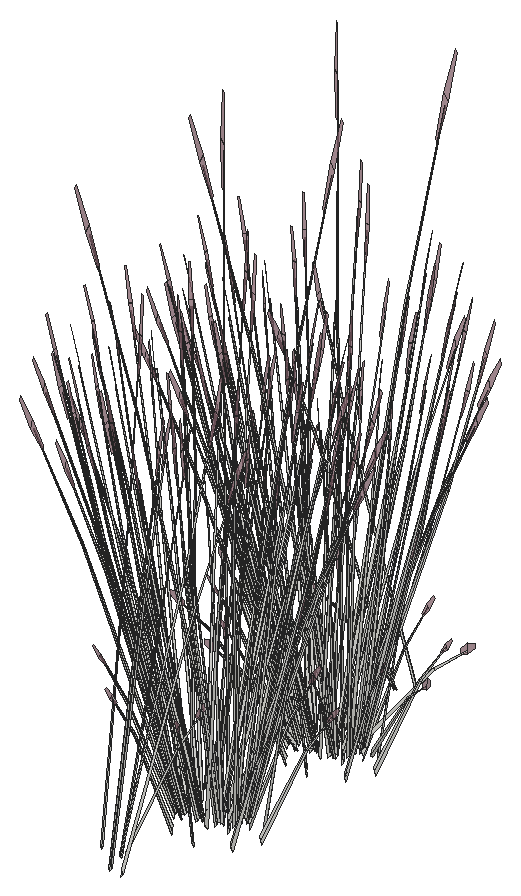
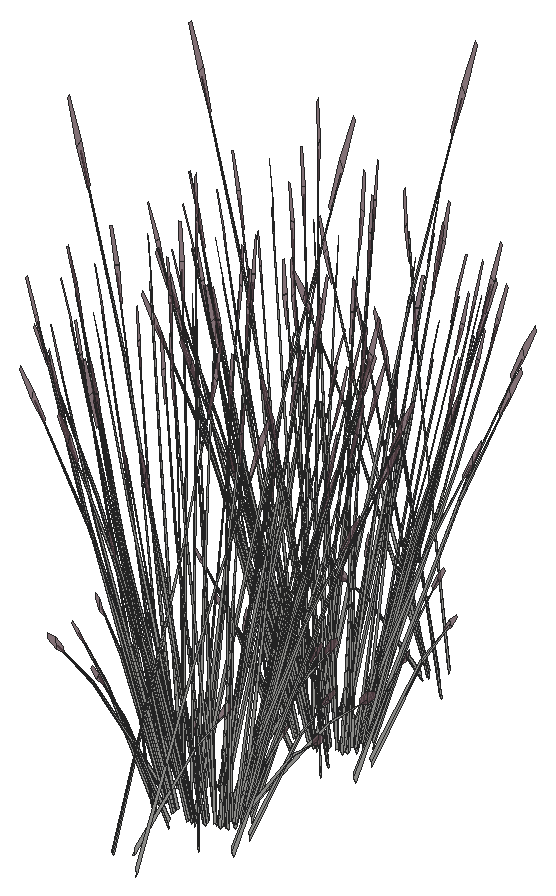
# SketchUp Ruby script. Lengths in inches.
U = 1.inch
M = Sketchup.active_model
def pt(a) = Geom::Point3d.new(a.map { |v| v * U })
def face(e, loops, mat)
  f = e.add_face(loops[0].map { |a| pt(a) })
  loops[1..].each { |l| e.add_face(l.map { |a| pt(a) }).erase! }
  f.material = f.back_material = mat if mat
  f
end
# faces: each face lists its corners as indices into pts; further lists are holes
def faces(e, pts, list, mat = nil) = list.each { |f| face(e, (f[0].is_a?(Array) ? f : [f]).map { |l| l.map { |i| pts[i] } }, mat) }
# xy, xz, yz: faces in a plane at the given z, y or x. An outline is a flat list of corners, or four numbers for a rectangle; further outlines are holes
def ring(l) = l.size == 4 ? [[l[0], l[1]], [l[2], l[1]], [l[2], l[3]], [l[0], l[3]]] : l.each_slice(2).to_a
def flat(e, list, mat, &to3) = list.each { |f| face(e, (f[0].is_a?(Array) ? f : [f]).map { |l| ring(l).map { |u, v| to3.(u, v) } }, mat) }
def xy(e, z, list, mat = nil) = flat(e, list, mat) { |x, y| [x, y, z] }
def xz(e, y, list, mat = nil) = flat(e, list, mat) { |x, z| [x, y, z] }
def yz(e, x, list, mat = nil) = flat(e, list, mat) { |y, z| [x, y, z] }
def lines(e, pts, list) = list.each { |a, b| e.add_line(pt(pts[a]), pt(pts[b])) }
# prism: a flat outline (further loops are holes) pulled along v
def prism(e, loops, v, mat = nil)
  f = face(e, loops, mat); d = Geom::Vector3d.new(v.map { |x| x * U })
  f.pushpull(f.normal.samedirection?(d) ? d.length : -d.length)
end
def box(e, o, s, mat = nil) = prism(e, [[o, [o[0] + s[0], o[1], o[2]], [o[0] + s[0], o[1] + s[1], o[2]], [o[0], o[1] + s[1], o[2]]]], [0, 0, s[2]], mat)
def at(x, y, z, deg = 0) = Geom::Transformation.translation(pt([x, y, z])) * Geom::Transformation.rotation(ORIGIN, Z_AXIS, deg.degrees)
def axes(o, x, y, z) = Geom::Transformation.new([*x, 0, *y, 0, *z, 0, *pt(o).to_a, 1])
def part(name) = M.definitions.add(name)
# library, detail: a bought-in or finely detailed component or shape, given as its bounding box
def library(name, o, s) = part(name).tap { |d| box(d.entities, o, s) }
def detail(e, o, s) = box(e.add_group.entities, o, s)
def put(e, d, t, mat = nil) = e.add_instance(d, t).tap { |i| i.material = mat if mat }
def group(e, t, mat = nil) = e.add_group.tap { |g| g.transformation = t; g.material = mat if mat }.entities
root = M.entities
M.materials.add("LightPink_Translucent").color = [144, 107, 117]
M.materials["LightPink_Translucent"].alpha = 0.75
c1 = part("blade")
p = [[2.15,0.21,22],[0,0.17,0],[0.09,0.45,0],[2.18,0.31,22],[2.29,0.31,22],[0.38,0.45,0],
  [2.48,0.24,33],[2.49,0.24,33],[2.48,0.22,33]]
faces(c1.entities,p,[[0,1,2,3],[4,5,2,3],[6,3,4,7],[8,0,3,6]])
c2 = part("seeds")
p = [[0.3,-0.1,1.38],[-0.01,-0.03,1.59],[-0.01,-0.03,0.03],[0.14,-0.07,-0.07],[0.29,-0.03,3],[0.15,0.01,3.11]]
faces(c2.entities,p,[[0,1,2,3],[1,0,4,5]],"LightPink_Translucent")
c3 = part("blade with seeds")
put(c3.entities,c1,at(0,0,0))
put(c3.entities,c2,axes([2.4,0.25,30.99],[1.5799,-0.05474,1.17369],[-0.12525,1.92788,0.29478],[-0.07173,-0.02425,1.56792]))
put(root,c3,axes([333.96,337.15,51.43],[-0.11542,-0.12546,1.51428],[0.53333,-0.10562,0.12244],[0.12054,0.19696,0.64734]))
put(root,c3,axes([333.45,338.05,52],[-0.15222,0.30049,-0.31292],[-0.44409,-0.08764,0.40398],[0.04072,0.12098,0.77298]))
put(root,c3,axes([332.49,337.47,52.72],[-0.01314,0.36145,-0.69681],[-0.55324,-0.02428,0.08409],[-0.05838,0.15313,0.9857]))
put(root,c3,axes([333.02,337.21,51.43],[-0.01236,-0.14998,1.51428],[0.53562,0.09949,0.12244],[-0.03313,0.21373,0.64734]))
put(root,c3,axes([333.5,337.78,52.4],[0.24099,0.31773,-0.62776],[-0.49607,0.17707,0.07576],[0.05635,0.15352,0.88802]))
put(root,c3,axes([333.14,338.58,52.17],[0.064,0.06292,1.54581],[0.51651,0.02472,-0.24447],[0.05194,0.13877,0.12397]))
put(root,c3,axes([332.69,344.625,51.43],[0.11542,0.12546,1.51428],[-0.53333,0.10562,0.12244],[-0.12054,-0.19696,0.64734]))
put(root,c3,axes([334.11,344.72,52.4],[-0.24099,-0.31773,-0.62776],[0.49607,-0.17707,0.07576],[-0.05635,-0.15352,0.88802]))
put(root,c3,axes([332.31,337.98,50.97],[0.01109,-0.20172,1.3638],[0.49896,0.10655,0.18846],[-0.04323,0.21498,0.64398]))
put(root,c3,axes([335.12,345.03,52.4],[0.01314,-0.36145,-0.62776],[0.55324,0.02428,0.07576],[0.05838,-0.15313,0.88802]))
put(root,c3,axes([334.16,344.45,52],[0.15222,-0.30049,-0.31292],[0.44409,0.08764,0.40398],[-0.04072,-0.12098,0.77298]))
put(root,c3,axes([334.5,344.85,51.43],[-0.09401,0.13431,1.51428],[-0.3944,-0.27795,0.12244],[0.17792,-0.17323,0.64734]))
put(root,c3,axes([333.93,344.66,52.14],[-0.49634,-0.09796,-0.45151],[0.17013,-0.33585,-0.34973],[-0.04551,-0.13522,0.86392]))
put(root,c3,axes([334.24,343.82,50.44],[0.06477,0.22786,1.01491],[-0.35932,-0.1262,0.74569],[0.03867,-0.11667,0.22354]))
put(root,c3,axes([335.01,344.91,52.14],[-0.36145,-0.26255,-0.45151],[0.38183,-0.22994,-0.34973],[0.055,-0.1334,0.86392]))
put(root,c3,axes([334.36,344.64,52.45],[-0.49409,0.18193,-0.10745],[-0.24281,-0.32289,-0.59638],[-0.06519,-0.13607,0.90619]))
put(root,c3,axes([335.38,345.05,52.45],[-0.55492,-0.01936,-0.10745],[0.01517,-0.36657,-0.59638],[0.03855,-0.14118,0.90619]))
put(root,c3,axes([335.35,344.8125,52],[0.34164,-0.20573,-0.31292],[0.3234,0.23491,0.40398],[0.04921,-0.11936,0.77298]))
put(root,c3,axes([332.39,344.09,50.44],[0.26338,0.136,1.01491],[-0.38358,0.08175,0.74569],[-0.08207,-0.10452,0.22354]))
put(root,c3,axes([333.03,344.81,52.4],[-0.43054,-0.18887,-0.62776],[0.30598,-0.33097,0.07576],[-0.15599,-0.11277,0.88802]))
put(root,c3,axes([332.88,344.56,52],[-0.07798,-0.31474,-0.31292],[0.44579,-0.08311,0.40398],[-0.11974,-0.09019,0.77298]))
put(root,c3,axes([331.92,345.02,51.43],[0.18755,0.06732,1.51428],[-0.38813,0.28243,0.12244],[-0.24191,-0.12741,0.64734]))
put(root,c3,axes([332.83,344.82,52.14],[-0.49824,0.09289,-0.45151],[-0.08716,-0.35177,-0.34973],[-0.13382,-0.10081,0.86392]))
put(root,c3,axes([335.77,345.66,52.4],[0.26374,-0.30832,-0.62776],[0.46217,0.21911,0.07576],[0.15748,-0.11171,0.88802]))
put(root,c3,axes([335.76,345.52,52.14],[-0.12971,-0.3568,-0.45151],[0.49122,-0.06241,-0.34973],[0.14077,-0.09583,0.86392]))
put(root,c3,axes([335.99,345.77,52.45],[-0.46706,-0.21546,-0.10745],[0.26908,-0.31203,-0.59638],[0.13196,-0.10846,0.90619]))
put(root,c3,axes([334.06,346.95,50.9375],[0.43633,0.15757,1.33654],[-0.42745,0.33945,0.52853],[-0.19146,-0.20119,1.12046]))
put(root,c3,axes([336.36,344.81,50.44],[-0.16818,0.19891,1.01491],[-0.14456,-0.26725,0.74569],[0.1389,-0.06697,0.22354]))
put(root,c3,axes([336.12,345.55,52],[0.43951,-0.05584,-0.31292],[0.11606,0.31924,0.40398],[0.12595,-0.08575,0.77298]))
put(root,c3,axes([331.85,345.11,52],[-0.28729,-0.24465,-0.31292],[0.32804,-0.23159,0.40398],[-0.16667,-0.03524,0.77298]))
put(root,c3,axes([332.15,345.28,52.4],[-0.50473,-0.00941,-0.62776],[0.0339,-0.39618,0.07576],[-0.21383,-0.04181,0.88802]))
put(root,c3,axes([331.98,345.36,52.14],[-0.36663,0.25884,-0.45151],[-0.32109,-0.27343,-0.34973],[-0.18628,-0.03938,0.86392]))
put(root,c3,axes([331.16,345.7,50.44],[0.32236,-0.02796,1.01491],[-0.20448,0.24636,0.74569],[-0.1593,-0.03696,0.22354]))
put(root,c3,axes([332.18,345.09,52.45],[-0.02704,0.39739,-0.10745],[-0.51189,-0.01086,-0.59638],[-0.19715,-0.0276,0.90619]))
put(root,c3,axes([336.01,346.61,52.45],[-0.25405,-0.35383,-0.10745],[0.45089,-0.17388,-0.59638],[0.19001,-0.04668,0.90619]))
put(root,c3,axes([335.98,346.31,52.14],[0.13679,-0.35544,-0.45151],[0.46898,0.12183,-0.34973],[0.18882,-0.03259,0.86392]))
put(root,c3,axes([331.52,345.63,51.43],[0.20943,-0.00885,1.51428],[-0.13893,0.38357,0.12244],[-0.29846,-0.02372,0.64734]))
put(root,c3,axes([335.9,346.4375,52.4],[0.44368,-0.17257,-0.62776],[0.24726,0.35524,0.07576],[0.21437,-0.04035,0.88802]))
put(root,c3,axes([336.27,346.47,52],[0.41962,0.10901,-0.31292],[-0.12239,0.31802,0.40398],[0.16894,-0.02916,0.77298]))
put(root,c3,axes([331.34,345.96,52],[-0.41962,-0.10901,-0.31292],[0.12239,-0.31802,0.40398],[-0.16894,0.02916,0.77298]))
put(root,c3,axes([335.13,346.08,51.43],[-0.20943,0.00885,1.51428],[0.13893,-0.38357,0.12244],[0.29846,0.02372,0.64734]))
put(root,c3,axes([332.62,345.91,50.95],[0.14352,-0.05653,1.56454],[0.04949,0.39467,0.12244],[-0.31087,0.05237,0.55918]))
put(root,c3,axes([337.16,346.53,50.44],[-0.31197,0.06451,1.01491],[0.14684,-0.26661,0.74569],[0.1655,0.01824,0.22354]))
put(root,c3,axes([331.63,346.125,52.14],[-0.13679,0.35544,-0.45151],[-0.46898,-0.12183,-0.34973],[-0.18882,0.03259,0.86392]))
put(root,c3,axes([331.61,345.82,52.45],[0.25405,0.35383,-0.10745],[-0.45089,0.17388,-0.59638],[-0.19001,0.04668,0.90619]))
put(root,c3,axes([336.62,347.36,51.47],[-0.09664,-0.32847,-0.03085],[0.45676,-0.07551,-0.13989],[0.09538,0.02082,0.4614]))
put(root,c3,axes([335.4375,347.35,52.45],[0.02704,-0.39739,-0.10745],[0.51189,0.01086,-0.59638],[0.19715,0.0276,0.90619]))
put(root,c3,axes([331.61,346.31,51.43],[0.17519,-0.08265,1.51428],[0.14749,0.38193,0.12244],[-0.27504,0.08632,0.64734]))
put(root,c3,axes([335.46,347.16,52.4],[0.50473,0.00941,-0.62776],[-0.0339,0.39618,0.07576],[0.21383,0.04181,0.88802]))
put(root,c3,axes([330.7,347.65,50.44],[0.21042,-0.1771,1.01491],[0.08303,0.28036,0.74569],[-0.15207,0.0502,0.22354]))
put(root,c3,axes([335.77,347.32,52],[0.28729,0.24465,-0.31292],[-0.32804,0.23159,0.40398],[0.16667,0.03524,0.77298]))
put(root,c3,axes([331.49,346.88,52],[-0.43951,0.05584,-0.31292],[-0.11606,-0.31924,0.40398],[-0.12595,0.08575,0.77298]))
put(root,c3,axes([334.73,346.69,51.43],[-0.18755,-0.06732,1.51428],[0.38813,-0.28243,0.12244],[0.24191,0.12741,0.64734]))
put(root,c3,axes([334.77,345.81,51.95],[-0.4363,-0.20303,1.22187],[0.46069,-0.31611,0.5272],[0.14077,0.1905,1.18105]))
put(root,c3,axes([331.625,346.66,52.45],[0.46706,0.21546,-0.10745],[-0.26908,0.31203,-0.59638],[-0.13196,0.10846,0.90619]))
put(root,c3,axes([335.43,347.46,50.44],[-0.28429,-0.11236,1.01491],[0.36709,-0.11416,0.74569],[0.09901,0.0967,0.22354]))
put(root,c3,axes([334.43,347.78,52.45],[0.30087,-0.33447,-0.10745],[0.43572,0.19269,-0.59638],[0.15146,0.0945,0.90619]))
put(root,c3,axes([332.25,346.57,51.43],[0.12611,-0.12006,1.51428],[0.31843,0.32408,0.12244],[-0.2184,0.14759,0.64734]))
put(root,c3,axes([331.86,346.92,52.14],[0.12971,0.3568,-0.45151],[-0.49122,0.06241,-0.34973],[-0.14077,0.09583,0.86392]))
put(root,c3,axes([334.74,346.19,50.51],[-0.01379,-0.36791,1.24828],[0.62424,0.09537,0.52853],[-0.14764,0.20132,1.17828]))
put(root,c3,axes([334.79,347.61,52.14],[0.49824,-0.09289,-0.45151],[0.08716,0.35177,-0.34973],[0.13382,0.10081,0.86392]))
put(root,c3,axes([332.16,346.86,51.43],[0.09401,-0.13431,1.51428],[0.3944,0.27795,0.12244],[-0.17792,0.17323,0.64734]))
put(root,c3,axes([332.27,347.62,52],[-0.34164,0.20573,-0.31292],[-0.3234,-0.23491,0.40398],[-0.04921,0.11936,0.77298]))
put(root,c3,axes([333.25,347.79,52.45],[0.49409,-0.18193,-0.10745],[0.24281,0.32289,-0.59638],[0.06519,0.13607,0.90619]))
put(root,c3,axes([332.48,348.42,50.44],[-0.01307,-0.23234,1.01491],[0.32652,0.16572,0.74569],[-0.06422,0.11074,0.22354]))
put(root,c3,axes([332.61,347.52,52.42],[0.36145,0.26255,-0.50118],[-0.38183,0.22994,-0.3882],[-0.055,0.1334,0.95895]))
put(root,c3,axes([333.68,347.78,52.14],[0.49634,0.09796,-0.45151],[-0.17013,0.33585,-0.34973],[0.04551,0.13522,0.86392]))
put(root,c3,axes([333.96,347.08,51.43],[-0.11542,-0.12546,1.51428],[0.53333,-0.10562,0.12244],[0.12054,0.19696,0.64734]))
put(root,c3,axes([333.45,347.98,52],[-0.15222,0.30049,-0.31292],[-0.44409,-0.08764,0.40398],[0.04072,0.12098,0.77298]))
put(root,c3,axes([332.49,347.4,52.72],[-0.01314,0.36145,-0.69681],[-0.55324,-0.02428,0.08409],[-0.05838,0.15313,0.9857]))
put(root,c3,axes([333.02,347.15,51.43],[-0.01236,-0.14998,1.51428],[0.53562,0.09949,0.12244],[-0.03313,0.21373,0.64734]))
put(root,c3,axes([333.5,347.71,52.4],[0.24099,0.31773,-0.62776],[-0.49607,0.17707,0.07576],[0.05635,0.15352,0.88802]))
put(root,c3,axes([332.31,347.91,50.97],[0.01109,-0.20172,1.3638],[0.49896,0.10655,0.18846],[-0.04323,0.21498,0.64398]))
put(root,c3,axes([332.69,355.35,51.43],[0.11542,0.12546,1.51428],[-0.53333,0.10562,0.12244],[-0.12054,-0.19696,0.64734]))
put(root,c3,axes([333.57,354.52,52.17],[-0.07723,-0.05479,1.54581],[-0.51538,0.03473,-0.24447],[-0.08225,-0.13104,0.12397]))
put(root,c3,axes([334.11,355.44,52.4],[-0.24099,-0.31773,-0.62776],[0.49607,-0.17707,0.07576],[-0.05635,-0.15352,0.88802]))
put(root,c3,axes([335.12,355.75,52.4],[0.01314,-0.36145,-0.62776],[0.55324,0.02428,0.07576],[0.05838,-0.15313,0.88802]))
put(root,c3,axes([335.89,355.1875,52.17],[-0.00487,-0.07777,1.54581],[-0.41166,-0.22476,-0.24447],[0.06364,-0.13625,0.12397]))
put(root,c3,axes([334.16,355.17,52],[0.15222,-0.30049,-0.31292],[0.44409,0.08764,0.40398],[-0.04072,-0.12098,0.77298]))
put(root,c3,axes([334.5,355.57,51.43],[-0.09401,0.13431,1.51428],[-0.3944,-0.27795,0.12244],[0.17792,-0.17323,0.64734]))
put(root,c3,axes([333.93,355.38,52.14],[-0.49634,-0.09796,-0.45151],[0.17013,-0.33585,-0.34973],[-0.04551,-0.13522,0.86392]))
put(root,c3,axes([334.24,354.54,50.44],[0.06477,0.22786,1.01491],[-0.35932,-0.1262,0.74569],[0.03867,-0.11667,0.22354]))
put(root,c3,axes([335.01,355.63,52.14],[-0.36145,-0.26255,-0.45151],[0.38183,-0.22994,-0.34973],[0.055,-0.1334,0.86392]))
put(root,c3,axes([334.36,355.36,52.45],[-0.49409,0.18193,-0.10745],[-0.24281,-0.32289,-0.59638],[-0.06519,-0.13607,0.90619]))
put(root,c3,axes([335.38,355.77,52.45],[-0.55492,-0.01936,-0.10745],[0.01517,-0.36657,-0.59638],[0.03855,-0.14118,0.90619]))
put(root,c3,axes([335.35,355.54,52],[0.34164,-0.20573,-0.31292],[0.3234,0.23491,0.40398],[0.04921,-0.11936,0.77298]))
put(root,c3,axes([332.39,354.8125,50.44],[0.26338,0.136,1.01491],[-0.38358,0.08175,0.74569],[-0.08207,-0.10452,0.22354]))
put(root,c3,axes([333.03,355.53,52.4],[-0.43054,-0.18887,-0.62776],[0.30598,-0.33097,0.07576],[-0.15599,-0.11277,0.88802]))
put(root,c3,axes([332.88,355.28,52],[-0.07798,-0.31474,-0.31292],[0.44579,-0.08311,0.40398],[-0.11974,-0.09019,0.77298]))
put(root,c3,axes([331.92,355.74,51.43],[0.18755,0.06732,1.51428],[-0.38813,0.28243,0.12244],[-0.24191,-0.12741,0.64734]))
put(root,c3,axes([332.83,355.54,52.14],[-0.49824,0.09289,-0.45151],[-0.08716,-0.35177,-0.34973],[-0.13382,-0.10081,0.86392]))
put(root,c3,axes([335.77,356.38,52.4],[0.26374,-0.30832,-0.62776],[0.46217,0.21911,0.07576],[0.15748,-0.11171,0.88802]))
put(root,c3,axes([335.76,356.24,52.14],[-0.12971,-0.3568,-0.45151],[0.49122,-0.06241,-0.34973],[0.14077,-0.09583,0.86392]))
put(root,c3,axes([331.88,355.12,52.17],[-0.10864,-0.00276,1.54581],[-0.34587,0.27582,-0.24447],[-0.18454,-0.05636,0.12397]))
put(root,c3,axes([335.99,356.49,52.45],[-0.46706,-0.21546,-0.10745],[0.26908,-0.31203,-0.59638],[0.13196,-0.10846,0.90619]))
put(root,c3,axes([334.06,357.67,50.9375],[0.43633,0.15757,1.33654],[-0.42745,0.33945,0.52853],[-0.19146,-0.20119,1.12046]))
put(root,c3,axes([336.36,355.53,50.44],[-0.16818,0.19891,1.01491],[-0.14456,-0.26725,0.74569],[0.1389,-0.06697,0.22354]))
put(root,c3,axes([336.12,356.27,52],[0.43951,-0.05584,-0.31292],[0.11606,0.31924,0.40398],[0.12595,-0.08575,0.77298]))
put(root,c3,axes([331.85,355.84,52],[-0.28729,-0.24465,-0.31292],[0.32804,-0.23159,0.40398],[-0.16667,-0.03524,0.77298]))
put(root,c3,axes([332.15,356,52.4],[-0.50473,-0.00941,-0.62776],[0.0339,-0.39618,0.07576],[-0.21383,-0.04181,0.88802]))
put(root,c3,axes([337.39,356.78,52.17],[0.07006,-0.05952,1.54581],[-0.08968,-0.3651,-0.24447],[0.1758,-0.06922,0.12397]))
put(root,c3,axes([331.98,356.08,52.14],[-0.36663,0.25884,-0.45151],[-0.32109,-0.27343,-0.34973],[-0.18628,-0.03938,0.86392]))
put(root,c3,axes([331.16,356.42,50.44],[0.32236,-0.02796,1.01491],[-0.20448,0.24636,0.74569],[-0.1593,-0.03696,0.22354]))
put(root,c3,axes([332.18,355.81,52.45],[-0.02704,0.39739,-0.10745],[-0.51189,-0.01086,-0.59638],[-0.19715,-0.0276,0.90619]))
put(root,c3,axes([336.01,357.33,52.45],[-0.25405,-0.35383,-0.10745],[0.45089,-0.17388,-0.59638],[0.19001,-0.04668,0.90619]))
put(root,c3,axes([335.98,357.03,52.14],[0.13679,-0.35544,-0.45151],[0.46898,0.12183,-0.34973],[0.18882,-0.03259,0.86392]))
put(root,c3,axes([331.52,356.36,51.43],[0.20943,-0.00885,1.51428],[-0.13893,0.38357,0.12244],[-0.29846,-0.02372,0.64734]))
put(root,c3,axes([335.9,357.16,52.4],[0.44368,-0.17257,-0.62776],[0.24726,0.35524,0.07576],[0.21437,-0.04035,0.88802]))
put(root,c3,axes([336.27,357.19,52],[0.41962,0.10901,-0.31292],[-0.12239,0.31802,0.40398],[0.16894,-0.02916,0.77298]))
put(root,c3,axes([331.34,356.69,52],[-0.41962,-0.10901,-0.31292],[0.12239,-0.31802,0.40398],[-0.16894,0.02916,0.77298]))
put(root,c3,axes([335.13,356.8,51.43],[-0.20943,0.00885,1.51428],[0.13893,-0.38357,0.12244],[0.29846,0.02372,0.64734]))
put(root,c3,axes([332.62,356.63,50.95],[0.14352,-0.05653,1.56454],[0.04949,0.39467,0.12244],[-0.31087,0.05237,0.55918]))
put(root,c3,axes([337.16,357.26,50.44],[-0.31197,0.06451,1.01491],[0.14684,-0.26661,0.74569],[0.1655,0.01824,0.22354]))
put(root,c3,axes([331.08,356.9,52.17],[-0.08245,0.05073,1.54581],[0.00701,0.37067,-0.24447],[-0.18899,0.0482,0.12397]))
put(root,c3,axes([331.63,356.85,52.14],[-0.13679,0.35544,-0.45151],[-0.46898,-0.12183,-0.34973],[-0.18882,0.03259,0.86392]))
put(root,c3,axes([331.61,356.54,52.45],[0.25405,0.35383,-0.10745],[-0.45089,0.17388,-0.59638],[-0.19001,0.04668,0.90619]))
put(root,c3,axes([336.62,358.08,51.47],[-0.09664,-0.32847,-0.03085],[0.45676,-0.07551,-0.13989],[0.09538,0.02082,0.4614]))
put(root,c3,axes([335.4375,358.07,52.45],[0.02704,-0.39739,-0.10745],[0.51189,0.01086,-0.59638],[0.19715,0.0276,0.90619]))
put(root,c3,axes([335.88,357.83,52.17],[0.10831,-0.00661,1.54581],[0.29709,-0.30358,-0.24447],[0.19266,0.04007,0.12397]))
put(root,c3,axes([331.61,357.03,51.43],[0.17519,-0.08265,1.51428],[0.14749,0.38193,0.12244],[-0.27504,0.08632,0.64734]))
put(root,c3,axes([335.46,357.88,52.4],[0.50473,0.00941,-0.62776],[-0.0339,0.39618,0.07576],[0.21383,0.04181,0.88802]))
put(root,c3,axes([330.7,358.37,50.44],[0.21042,-0.1771,1.01491],[0.08303,0.28036,0.74569],[-0.15207,0.0502,0.22354]))
put(root,c3,axes([335.77,358.04,52],[0.28729,0.24465,-0.31292],[-0.32804,0.23159,0.40398],[0.16667,0.03524,0.77298]))
put(root,c3,axes([331.49,357.6,52],[-0.43951,0.05584,-0.31292],[-0.11606,-0.31924,0.40398],[-0.12595,0.08575,0.77298]))
put(root,c3,axes([334.73,357.41,51.43],[-0.18755,-0.06732,1.51428],[0.38813,-0.28243,0.12244],[0.24191,0.12741,0.64734]))
put(root,c3,axes([334.77,356.53,51.95],[-0.4363,-0.20303,1.22187],[0.46069,-0.31611,0.5272],[0.14077,0.1905,1.18105]))
put(root,c3,axes([331.625,357.38,52.45],[0.46706,0.21546,-0.10745],[-0.26908,0.31203,-0.59638],[-0.13196,0.10846,0.90619]))
put(root,c3,axes([335.43,358.18,50.44],[-0.28429,-0.11236,1.01491],[0.36709,-0.11416,0.74569],[0.09901,0.0967,0.22354]))
put(root,c3,axes([334.43,358.5,52.45],[0.30087,-0.33447,-0.10745],[0.43572,0.19269,-0.59638],[0.15146,0.0945,0.90619]))
put(root,c3,axes([332.25,357.29,51.43],[0.12611,-0.12006,1.51428],[0.31843,0.32408,0.12244],[-0.2184,0.14759,0.64734]))
put(root,c3,axes([331.86,357.64,52.14],[0.12971,0.3568,-0.45151],[-0.49122,0.06241,-0.34973],[-0.14077,0.09583,0.86392]))
put(root,c3,axes([334.74,356.92,50.51],[-0.01379,-0.36791,1.24828],[0.62424,0.09537,0.52853],[-0.14764,0.20132,1.17828]))
put(root,c3,axes([334.79,358.34,52.14],[0.49824,-0.09289,-0.45151],[0.08716,0.35177,-0.34973],[0.13382,0.10081,0.86392]))
put(root,c3,axes([332.16,357.58,51.43],[0.09401,-0.13431,1.51428],[0.3944,0.27795,0.12244],[-0.17792,0.17323,0.64734]))
put(root,c3,axes([332.27,358.34,52],[-0.34164,0.20573,-0.31292],[-0.3234,-0.23491,0.40398],[-0.04921,0.11936,0.77298]))
put(root,c3,axes([331.09,358.28,52.17],[-0.01255,0.07733,1.54581],[0.35618,0.269,-0.24447],[-0.09325,0.12721,0.12397]))
put(root,c3,axes([333.25,358.51,52.45],[0.49409,-0.18193,-0.10745],[0.24281,0.32289,-0.59638],[0.06519,0.13607,0.90619]))
put(root,c3,axes([332.48,359.14,50.44],[-0.01307,-0.23234,1.01491],[0.32652,0.16572,0.74569],[-0.06422,0.11074,0.22354]))
put(root,c3,axes([332.61,358.24,52.42],[0.36145,0.26255,-0.50118],[-0.38183,0.22994,-0.3882],[-0.055,0.1334,0.95895]))
put(root,c3,axes([333.68,358.5,52.14],[0.49634,0.09796,-0.45151],[-0.17013,0.33585,-0.34973],[0.04551,0.13522,0.86392]))
put(root,c3,axes([333.96,357.81,51.43],[-0.11542,-0.12546,1.51428],[0.53333,-0.10562,0.12244],[0.12054,0.19696,0.64734]))
put(root,c3,axes([333.45,358.7,52],[-0.15222,0.30049,-0.31292],[-0.44409,-0.08764,0.40398],[0.04072,0.12098,0.77298]))
put(root,c3,axes([332.69,364.67,51.43],[0.11542,0.12546,1.51428],[-0.53333,0.10562,0.12244],[-0.12054,-0.19696,0.64734]))
put(root,c3,axes([333.57,363.84,52.17],[-0.07723,-0.05479,1.54581],[-0.51538,0.03473,-0.24447],[-0.08225,-0.13104,0.12397]))
put(root,c3,axes([332.49,358.125,52.72],[-0.01314,0.36145,-0.69681],[-0.55324,-0.02428,0.08409],[-0.05838,0.15313,0.9857]))
put(root,c3,axes([334.11,364.77,52.4],[-0.24099,-0.31773,-0.62776],[0.49607,-0.17707,0.07576],[-0.05635,-0.15352,0.88802]))
put(root,c3,axes([333.02,357.87,51.43],[-0.01236,-0.14998,1.51428],[0.53562,0.09949,0.12244],[-0.03313,0.21373,0.64734]))
put(root,c3,axes([333.5,358.43,52.4],[0.24099,0.31773,-0.62776],[-0.49607,0.17707,0.07576],[0.05635,0.15352,0.88802]))
